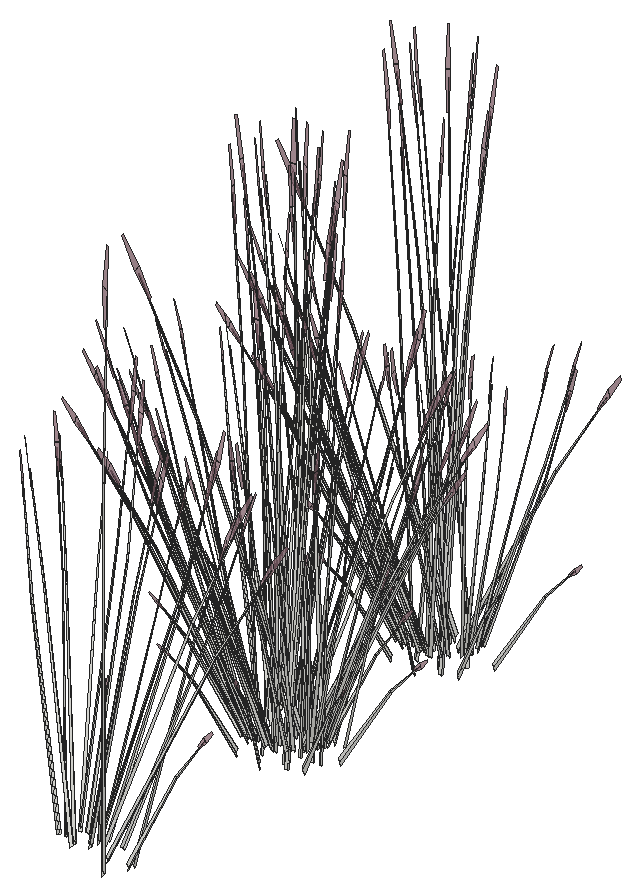
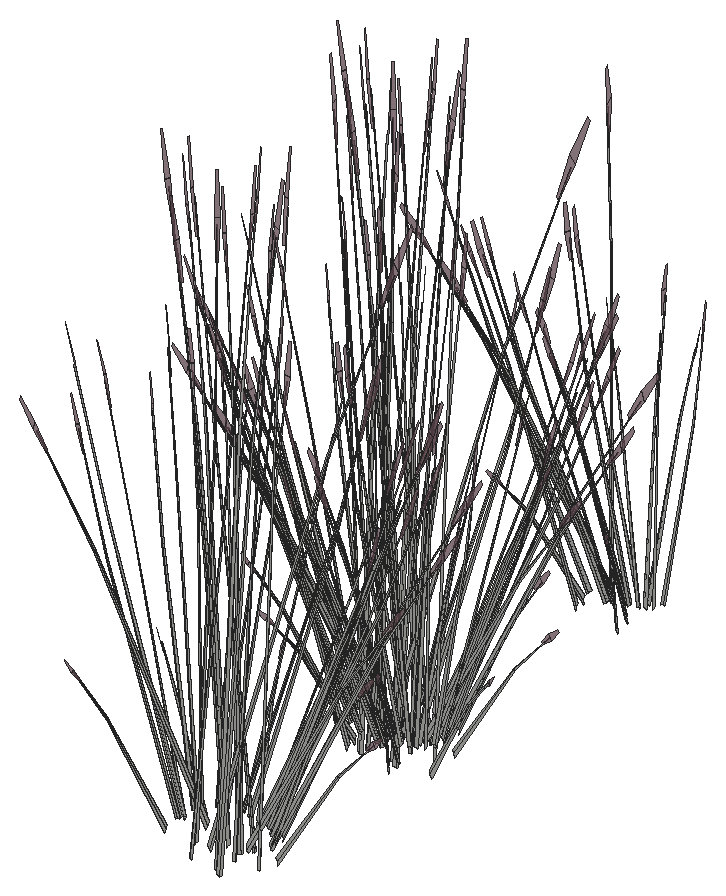
# SketchUp Ruby script. Lengths in inches.
U = 1.inch
M = Sketchup.active_model
def pt(a) = Geom::Point3d.new(a.map { |v| v * U })
def face(e, loops, mat)
  f = e.add_face(loops[0].map { |a| pt(a) })
  loops[1..].each { |l| e.add_face(l.map { |a| pt(a) }).erase! }
  f.material = f.back_material = mat if mat
  f
end
# faces: each face lists its corners as indices into pts; further lists are holes
def faces(e, pts, list, mat = nil) = list.each { |f| face(e, (f[0].is_a?(Array) ? f : [f]).map { |l| l.map { |i| pts[i] } }, mat) }
# xy, xz, yz: faces in a plane at the given z, y or x. An outline is a flat list of corners, or four numbers for a rectangle; further outlines are holes
def ring(l) = l.size == 4 ? [[l[0], l[1]], [l[2], l[1]], [l[2], l[3]], [l[0], l[3]]] : l.each_slice(2).to_a
def flat(e, list, mat, &to3) = list.each { |f| face(e, (f[0].is_a?(Array) ? f : [f]).map { |l| ring(l).map { |u, v| to3.(u, v) } }, mat) }
def xy(e, z, list, mat = nil) = flat(e, list, mat) { |x, y| [x, y, z] }
def xz(e, y, list, mat = nil) = flat(e, list, mat) { |x, z| [x, y, z] }
def yz(e, x, list, mat = nil) = flat(e, list, mat) { |y, z| [x, y, z] }
def lines(e, pts, list) = list.each { |a, b| e.add_line(pt(pts[a]), pt(pts[b])) }
# prism: a flat outline (further loops are holes) pulled along v
def prism(e, loops, v, mat = nil)
  f = face(e, loops, mat); d = Geom::Vector3d.new(v.map { |x| x * U })
  f.pushpull(f.normal.samedirection?(d) ? d.length : -d.length)
end
def box(e, o, s, mat = nil) = prism(e, [[o, [o[0] + s[0], o[1], o[2]], [o[0] + s[0], o[1] + s[1], o[2]], [o[0], o[1] + s[1], o[2]]]], [0, 0, s[2]], mat)
def at(x, y, z, deg = 0) = Geom::Transformation.translation(pt([x, y, z])) * Geom::Transformation.rotation(ORIGIN, Z_AXIS, deg.degrees)
def axes(o, x, y, z) = Geom::Transformation.new([*x, 0, *y, 0, *z, 0, *pt(o).to_a, 1])
def part(name) = M.definitions.add(name)
# library, detail: a bought-in or finely detailed component or shape, given as its bounding box
def library(name, o, s) = part(name).tap { |d| box(d.entities, o, s) }
def detail(e, o, s) = box(e.add_group.entities, o, s)
def put(e, d, t, mat = nil) = e.add_instance(d, t).tap { |i| i.material = mat if mat }
def group(e, t, mat = nil) = e.add_group.tap { |g| g.transformation = t; g.material = mat if mat }.entities
root = M.entities
M.materials.add("LightPink_Translucent").color = [144, 107, 117]
M.materials["LightPink_Translucent"].alpha = 0.75
c1 = part("blade")
p = [[2.15,0.21,22],[0,0.17,0],[0.09,0.45,0],[2.18,0.31,22],[2.29,0.31,22],[0.38,0.45,0],
  [2.48,0.24,33],[2.49,0.24,33],[2.48,0.22,33]]
faces(c1.entities,p,[[0,1,2,3],[4,5,2,3],[6,3,4,7],[8,0,3,6]])
c2 = part("seeds")
p = [[0.3,-0.1,1.38],[-0.01,-0.03,1.59],[-0.01,-0.03,0.03],[0.14,-0.07,-0.07],[0.29,-0.03,3],[0.15,0.01,3.11]]
faces(c2.entities,p,[[0,1,2,3],[1,0,4,5]],"LightPink_Translucent")
c3 = part("blade with seeds")
put(c3.entities,c1,at(0,0,0))
put(c3.entities,c2,axes([2.4,0.25,30.99],[1.5799,-0.05474,1.17369],[-0.12525,1.92788,0.29478],[-0.07173,-0.02425,1.56792]))
put(root,c3,axes([668.72,239.06,513.76],[-0.56631,0.0816,-0.29394],[-0.14954,-0.46647,0.37948],[-0.16229,0.12529,0.72609]))
put(root,c3,axes([672.9,238.78,513.22],[-0.24166,-0.09837,1.42242],[0.50011,-0.41269,0.11501],[0.3117,0.18617,0.60807]))
put(root,c3,axes([673.79,239.9,512.3],[-0.36631,-0.16417,0.95334],[0.47299,-0.16681,0.70045],[0.12758,0.1413,0.20998]))
put(root,c3,axes([669.7,238.6,513.22],[0.1625,-0.17544,1.42242],[0.41029,0.47354,0.11501],[-0.28141,0.21565,0.60807]))
put(root,c3,axes([669.1875,239.11,513.89],[0.16713,0.52135,-0.42412],[-0.63294,0.0912,-0.32852],[-0.18138,0.14003,0.81151]))
put(root,c3,axes([672.9,238.06,512.36],[-0.01777,-0.53759,1.17256],[0.80434,0.13935,0.49647],[-0.19024,0.29416,1.1068]))
put(root,c3,axes([672.96,240.13,513.89],[0.64198,-0.13573,-0.42412],[0.1123,0.514,-0.32852],[0.17243,0.1473,0.81151]))
put(root,c3,axes([673.85,240.65,512.21],[-0.4172,-0.01791,0.872],[0.27552,-0.38032,0.48145],[0.16481,0.13512,0.68401]))
put(root,c3,axes([669.58,239.03,513.22],[0.12114,-0.19625,1.42242],[0.50818,0.40613,0.11501],[-0.22925,0.25313,0.60807]))
put(root,c3,axes([669.72,240.14,513.76],[-0.4402,0.30062,-0.29394],[-0.41671,-0.34326,0.37948],[-0.0634,0.1744,0.72609]))
put(root,c3,axes([670,241.31,512.3],[-0.01684,-0.3395,0.95334],[0.42072,0.24214,0.70045],[-0.08274,0.16182,0.20998]))
put(root,c3,axes([670.16,240,514.15],[0.46573,0.38364,-0.47077],[-0.49199,0.33598,-0.36465],[-0.07086,0.19492,0.90078]))
put(root,c3,axes([671.54,240.37,513.89],[0.63954,0.14313,-0.42412],[-0.21921,0.49074,-0.32852],[0.05864,0.19758,0.81151]))
put(root,c3,axes([671.9,239.35,513.22],[-0.14872,-0.18332,1.42242],[0.6872,-0.15433,0.11501],[0.15531,0.28779,0.60807]))
put(root,c3,axes([671.25,240.67,513.76],[-0.19614,0.43908,-0.29394],[-0.57222,-0.12807,0.37948],[0.05247,0.17678,0.72609]))
put(root,c3,axes([670.01,239.82,514.43],[-0.01693,0.52814,-0.65454],[-0.71285,-0.03547,0.07899],[-0.07523,0.22375,0.92591]))
put(root,c3,axes([670.6875,239.45,513.22],[-0.01592,-0.21915,1.42242],[0.69015,0.14538,0.11501],[-0.04269,0.3123,0.60807]))
put(root,c3,axes([671.3,240.27,514.13],[0.31051,0.46426,-0.58968],[-0.63919,0.25873,0.07116],[0.07261,0.22432,0.83415]))
put(root,c3,axes([669.77,240.5625,512.79],[0.01429,-0.29475,1.28107],[0.64291,0.15569,0.17703],[-0.0557,0.31414,0.60492]))
put(root,c3,axes([670.27,257.61,513.22],[0.14872,0.18332,1.42242],[-0.6872,0.15433,0.11501],[-0.15531,-0.28779,0.60807]))
put(root,c3,axes([672.1,257.75,514.13],[-0.31051,-0.46426,-0.58968],[0.63919,-0.25873,0.07116],[-0.07261,-0.22432,0.83415]))
put(root,c3,axes([673.39,258.2,514.13],[0.01693,-0.52814,-0.58968],[0.71285,0.03547,0.07116],[0.07523,-0.22375,0.83415]))
put(root,c3,axes([672.16,257.35,513.76],[0.19614,-0.43908,-0.29394],[0.57222,0.12807,0.37948],[-0.05247,-0.17678,0.72609]))
put(root,c3,axes([672.59,257.93,513.22],[-0.12114,0.19625,1.42242],[-0.50818,-0.40613,0.11501],[0.22925,-0.25313,0.60807]))
put(root,c3,axes([671.87,257.65,513.89],[-0.63954,-0.14313,-0.42412],[0.21921,-0.49074,-0.32852],[-0.05864,-0.19758,0.81151]))
put(root,c3,axes([672.26,256.43,512.3],[0.08346,0.33295,0.95334],[-0.46298,-0.1844,0.70045],[0.04982,-0.17048,0.20998]))
put(root,c3,axes([673.25,258.03,513.89],[-0.46573,-0.38364,-0.42412],[0.49199,-0.33598,-0.32852],[0.07086,-0.19492,0.81151]))
put(root,c3,axes([673.69,257.88,513.76],[0.4402,-0.30062,-0.29394],[0.41671,0.34326,0.37948],[0.0634,-0.1744,0.72609]))
put(root,c3,axes([669.88,256.83,512.3],[0.33937,0.19872,0.95334],[-0.49424,0.11946,0.70045],[-0.10575,-0.15273,0.20998]))
put(root,c3,axes([670.7,257.88,514.13],[-0.55475,-0.27598,-0.58968],[0.39425,-0.48361,0.07116],[-0.20099,-0.16478,0.83415]))
put(root,c3,axes([670.51,257.51,513.76],[-0.10048,-0.4599,-0.29394],[0.5744,-0.12144,0.37948],[-0.15428,-0.13179,0.72609]))
put(root,c3,axes([669.27,258.18,513.22],[0.24166,0.09837,1.42242],[-0.50011,0.41269,0.11501],[-0.3117,-0.18617,0.60807]))
put(root,c3,axes([670.44,257.89,513.89],[-0.64198,0.13573,-0.42412],[-0.1123,-0.514,-0.32852],[-0.17243,-0.1473,0.81151]))
put(root,c3,axes([674.23,259.12,514.13],[0.33983,-0.45051,-0.58968],[0.59551,0.32017,0.07116],[0.20291,-0.16322,0.83415]))
put(root,c3,axes([674.21,258.91,513.89],[-0.16713,-0.52135,-0.42412],[0.63294,-0.0912,-0.32852],[0.18138,-0.14003,0.81151]))
put(root,c3,axes([672.03,261,512.76],[0.56221,0.23024,1.25546],[-0.55078,0.49601,0.49647],[-0.2467,-0.29398,1.05249]))
put(root,c3,axes([674.99,257.87,512.3],[-0.2167,0.29065,0.95334],[-0.18626,-0.3905,0.70045],[0.17898,-0.09785,0.20998]))
put(root,c3,axes([674.68,258.96,513.76],[0.56631,-0.0816,-0.29394],[0.14954,0.46647,0.37948],[0.16229,-0.12529,0.72609]))
put(root,c3,axes([669.18,258.32,513.76],[-0.37017,-0.35748,-0.29394],[0.42268,-0.3384,0.37948],[-0.21476,-0.05149,0.72609]))
put(root,c3,axes([669.57,258.5625,514.13],[-0.65035,-0.01375,-0.58968],[0.04368,-0.5789,0.07116],[-0.27552,-0.06109,0.83415]))
put(root,c3,axes([669.35,258.68,513.89],[-0.47241,0.37822,-0.42412],[-0.41372,-0.39954,-0.32852],[-0.24002,-0.05755,0.81151]))
put(root,c3,axes([668.29,259.18,512.3],[0.41536,-0.04086,0.95334],[-0.26347,0.35999,0.70045],[-0.20525,-0.054,0.20998]))
put(root,c3,axes([671.22,259.51,512.26],[-0.70648,0.03525,0.37133],[-0.06389,-0.58508,-0.17871],[0.12647,-0.0593,1.19224]))
put(root,c3,axes([669.4,259.9375,512.06],[0,0.57097,0.4121],[-0.72788,0,0],[0,-0.13004,1.30728]))
put(root,c3,axes([674.51,260.07,513.89],[0.17625,-0.51936,-0.42412],[0.60429,0.17802,-0.32852],[0.2433,-0.04762,0.81151]))
put(root,c3,axes([668.76,259.08,513.22],[0.26985,-0.01293,1.42242],[-0.17902,0.56047,0.11501],[-0.38456,-0.03467,0.60807]))
put(root,c3,axes([671.06,260.23,512.26],[-0.31565,0.51449,0.37133],[-0.65588,-0.24761,-0.17871],[0,-0.1186,1.19224]))
put(root,c3,axes([673.2,258.25,512.06],[-0.60889,-0.28548,0.4121],[0.36394,-0.51192,0],[0.13868,0.06502,1.30728]))
put(root,c3,axes([674.39,260.26,514.13],[0.57168,-0.25217,-0.58968],[0.3186,0.51908,0.07116],[0.27622,-0.05897,0.83415]))
put(root,c3,axes([670.89,258.51,512.05],[-0.18794,0.56744,0.14643],[-0.68774,-0.16058,0.29122],[0.1188,-0.00276,1.33138]))
put(root,c3,axes([672.07,259.27,512.26],[-0.39083,-0.47924,0.37133],[0.59199,-0.33747,-0.17871],[0.12647,0.0593,1.19224]))
put(root,c3,axes([670.83,261.43,512.05],[0.6991,-0.15154,0.14643],[0.17263,0.56398,0.29122],[-0.06235,-0.08217,1.33138]))
put(root,c3,axes([674.88,260.3,513.76],[0.54068,0.15928,-0.29394],[-0.1577,0.46469,0.37948],[0.21769,-0.04261,0.72609]))
put(root,c3,axes([668.52,259.5625,513.76],[-0.54068,-0.15928,-0.29394],[0.1577,-0.46469,0.37948],[-0.21769,0.04261,0.72609]))
put(root,c3,axes([672.97,258.54,512.05],[-0.6991,0.15154,0.14643],[-0.17263,-0.56398,0.29122],[0.06235,0.08217,1.33138]))
put(root,c3,axes([673.41,259.73,513.22],[-0.26985,0.01293,1.42242],[0.17902,-0.56047,0.11501],[0.38456,0.03467,0.60807]))
put(root,c3,axes([672.91,261.47,512.05],[0.18794,-0.56744,0.14643],[0.68774,0.16058,0.29122],[-0.1188,0.00276,1.33138]))
put(root,c3,axes([670.17,259.49,512.77],[0.18493,-0.0826,1.46963],[0.06377,0.5767,0.11501],[-0.40056,0.07652,0.52526]))
put(root,c3,axes([673.98,260.02,512.05],[-0.51116,-0.4159,0.14643],[0.51512,-0.4034,0.29122],[-0.05645,0.08494,1.33138]))
put(root,c3,axes([676.03,260.4,512.3],[-0.40197,0.09426,0.95334],[0.18921,-0.38956,0.70045],[0.21325,0.02666,0.20998]))
put(root,c3,axes([670.6,261.72,512.06],[0.60889,0.28548,0.4121],[-0.36394,0.51192,0],[-0.13868,-0.06502,1.30728]))
put(root,c3,axes([672.75,259.75,512.26],[0.31565,-0.51449,0.37133],[0.65588,0.24761,-0.17871],[0,0.1186,1.19224]))
put(root,c3,axes([668.89,259.8,513.89],[-0.17625,0.51936,-0.42412],[-0.60429,-0.17802,-0.32852],[-0.2433,0.04762,0.81151]))
put(root,c3,axes([675.33,261.6,513.26],[-0.12452,-0.47997,-0.02898],[0.58854,-0.11034,-0.1314],[0.1229,0.03043,0.43341]))
put(root,c3,axes([674.4,260.03,512.06],[0,-0.57097,0.4121],[0.72788,0,0],[0,0.13004,1.30728]))
put(root,c3,axes([672.58,260.46,512.26],[0.70648,-0.03525,0.37133],[0.06389,0.58508,-0.17871],[-0.12647,0.0593,1.19224]))
put(root,c3,axes([668.875,260.07,513.22],[0.22574,-0.12077,1.42242],[0.19004,0.55807,0.11501],[-0.35439,0.12613,0.60807]))
put(root,c3,axes([673.83,261.31,514.13],[0.65035,0.01375,-0.58968],[-0.04368,0.5789,0.07116],[0.27552,0.06109,0.83415]))
put(root,c3,axes([673.1,261.77,512.06],[0.60889,-0.28548,0.4121],[0.36394,0.51192,0],[-0.13868,0.06502,1.30728]))
put(root,c3,axes([667.7,262.02,512.3],[0.27113,-0.25877,0.95334],[0.10699,0.40966,0.70045],[-0.19594,0.07335,0.20998]))
put(root,c3,axes([674.23,261.54,513.76],[0.37017,0.35748,-0.29394],[-0.42268,0.3384,0.37948],[0.21476,0.05149,0.72609]))
put(root,c3,axes([668.72,260.9,513.76],[-0.56631,0.0816,-0.29394],[-0.14954,-0.46647,0.37948],[-0.16229,0.12529,0.72609]))
put(root,c3,axes([672.9,260.63,513.22],[-0.24166,-0.09837,1.42242],[0.50011,-0.41269,0.11501],[0.3117,0.18617,0.60807]))
put(root,c3,axes([673.79,261.75,512.3],[-0.36631,-0.16417,0.95334],[0.47299,-0.16681,0.70045],[0.12758,0.1413,0.20998]))
put(root,c3,axes([669.7,260.44,513.22],[0.1625,-0.17544,1.42242],[0.41029,0.47354,0.11501],[-0.28141,0.21565,0.60807]))
put(root,c3,axes([669.1875,260.96,513.89],[0.16713,0.52135,-0.42412],[-0.63294,0.0912,-0.32852],[-0.18138,0.14003,0.81151]))
put(root,c3,axes([672.9,259.9,512.36],[-0.01777,-0.53759,1.17256],[0.80434,0.13935,0.49647],[-0.19024,0.29416,1.1068]))
put(root,c3,axes([672.96,261.97,513.89],[0.64198,-0.13573,-0.42412],[0.1123,0.514,-0.32852],[0.17243,0.1473,0.81151]))
put(root,c3,axes([673.85,262.5,512.21],[-0.4172,-0.01791,0.872],[0.27552,-0.38032,0.48145],[0.16481,0.13512,0.68401]))
put(root,c3,axes([669.58,260.875,513.22],[0.12114,-0.19625,1.42242],[0.50818,0.40613,0.11501],[-0.22925,0.25313,0.60807]))
put(root,c3,axes([669.72,261.98,513.76],[-0.4402,0.30062,-0.29394],[-0.41671,-0.34326,0.37948],[-0.0634,0.1744,0.72609]))
put(root,c3,axes([670,263.15,512.3],[-0.01684,-0.3395,0.95334],[0.42072,0.24214,0.70045],[-0.08274,0.16182,0.20998]))
put(root,c3,axes([670.16,261.84,514.15],[0.46573,0.38364,-0.47077],[-0.49199,0.33598,-0.36465],[-0.07086,0.19492,0.90078]))
put(root,c3,axes([671.54,262.21,513.89],[0.63954,0.14313,-0.42412],[-0.21921,0.49074,-0.32852],[0.05864,0.19758,0.81151]))
put(root,c3,axes([671.9,261.2,513.22],[-0.14872,-0.18332,1.42242],[0.6872,-0.15433,0.11501],[0.15531,0.28779,0.60807]))
put(root,c3,axes([671.25,262.51,513.76],[-0.19614,0.43908,-0.29394],[-0.57222,-0.12807,0.37948],[0.05247,0.17678,0.72609]))
put(root,c3,axes([670.01,261.67,514.43],[-0.01693,0.52814,-0.65454],[-0.71285,-0.03547,0.07899],[-0.07523,0.22375,0.92591]))
put(root,c3,axes([670.6875,261.29,513.22],[-0.01592,-0.21915,1.42242],[0.69015,0.14538,0.11501],[-0.04269,0.3123,0.60807]))
put(root,c3,axes([671.3,262.12,514.13],[0.31051,0.46426,-0.58968],[-0.63919,0.25873,0.07116],[0.07261,0.22432,0.83415]))
put(root,c3,axes([669.77,262.41,512.79],[0.01429,-0.29475,1.28107],[0.64291,0.15569,0.17703],[-0.0557,0.31414,0.60492]))
put(root,c3,axes([670.27,274.47,513.22],[0.14872,0.18332,1.42242],[-0.6872,0.15433,0.11501],[-0.15531,-0.28779,0.60807]))
put(root,c3,axes([672.1,274.61,514.13],[-0.31051,-0.46426,-0.58968],[0.63919,-0.25873,0.07116],[-0.07261,-0.22432,0.83415]))
put(root,c3,axes([673.39,275.06,514.13],[0.01693,-0.52814,-0.58968],[0.71285,0.03547,0.07116],[0.07523,-0.22375,0.83415]))
put(root,c3,axes([672.16,274.21,513.76],[0.19614,-0.43908,-0.29394],[0.57222,0.12807,0.37948],[-0.05247,-0.17678,0.72609]))
put(root,c3,axes([672.59,274.79,513.22],[-0.12114,0.19625,1.42242],[-0.50818,-0.40613,0.11501],[0.22925,-0.25313,0.60807]))
put(root,c3,axes([671.87,274.51,513.89],[-0.63954,-0.14313,-0.42412],[0.21921,-0.49074,-0.32852],[-0.05864,-0.19758,0.81151]))
put(root,c3,axes([672.26,273.28,512.3],[0.08346,0.33295,0.95334],[-0.46298,-0.1844,0.70045],[0.04982,-0.17048,0.20998]))
put(root,c3,axes([673.25,274.89,513.89],[-0.46573,-0.38364,-0.42412],[0.49199,-0.33598,-0.32852],[0.07086,-0.19492,0.81151]))
put(root,c3,axes([673.69,274.74,513.76],[0.4402,-0.30062,-0.29394],[0.41671,0.34326,0.37948],[0.0634,-0.1744,0.72609]))
put(root,c3,axes([669.88,273.68,512.3],[0.33937,0.19872,0.95334],[-0.49424,0.11946,0.70045],[-0.10575,-0.15273,0.20998]))
put(root,c3,axes([670.7,274.74,514.13],[-0.55475,-0.27598,-0.58968],[0.39425,-0.48361,0.07116],[-0.20099,-0.16478,0.83415]))
put(root,c3,axes([670.51,274.37,513.76],[-0.10048,-0.4599,-0.29394],[0.5744,-0.12144,0.37948],[-0.15428,-0.13179,0.72609]))
put(root,c3,axes([669.27,275.04,513.22],[0.24166,0.09837,1.42242],[-0.50011,0.41269,0.11501],[-0.3117,-0.18617,0.60807]))
put(root,c3,axes([670.44,274.75,513.89],[-0.64198,0.13573,-0.42412],[-0.1123,-0.514,-0.32852],[-0.17243,-0.1473,0.81151]))
put(root,c3,axes([674.23,275.98,514.13],[0.33983,-0.45051,-0.58968],[0.59551,0.32017,0.07116],[0.20291,-0.16322,0.83415]))
put(root,c3,axes([674.21,275.77,513.89],[-0.16713,-0.52135,-0.42412],[0.63294,-0.0912,-0.32852],[0.18138,-0.14003,0.81151]))
put(root,c3,axes([672.03,277.86,512.76],[0.56221,0.23024,1.25546],[-0.55078,0.49601,0.49647],[-0.2467,-0.29398,1.05249]))
put(root,c3,axes([674.99,274.73,512.3],[-0.2167,0.29065,0.95334],[-0.18626,-0.3905,0.70045],[0.17898,-0.09785,0.20998]))
put(root,c3,axes([674.68,275.82,513.76],[0.56631,-0.0816,-0.29394],[0.14954,0.46647,0.37948],[0.16229,-0.12529,0.72609]))
put(root,c3,axes([669.18,275.18,513.76],[-0.37017,-0.35748,-0.29394],[0.42268,-0.3384,0.37948],[-0.21476,-0.05149,0.72609]))
put(root,c3,axes([669.57,275.42,514.13],[-0.65035,-0.01375,-0.58968],[0.04368,-0.5789,0.07116],[-0.27552,-0.06109,0.83415]))
put(root,c3,axes([669.35,275.54,513.89],[-0.47241,0.37822,-0.42412],[-0.41372,-0.39954,-0.32852],[-0.24002,-0.05755,0.81151]))
put(root,c3,axes([668.29,276.04,512.3],[0.41536,-0.04086,0.95334],[-0.26347,0.35999,0.70045],[-0.20525,-0.054,0.20998]))
put(root,c3,axes([671.22,276.37,512.26],[-0.70648,0.03525,0.37133],[-0.06389,-0.58508,-0.17871],[0.12647,-0.0593,1.19224]))
put(root,c3,axes([669.4,276.8,512.06],[0,0.57097,0.4121],[-0.72788,0,0],[0,-0.13004,1.30728]))
put(root,c3,axes([674.51,276.93,513.89],[0.17625,-0.51936,-0.42412],[0.60429,0.17802,-0.32852],[0.2433,-0.04762,0.81151]))
put(root,c3,axes([668.76,275.94,513.22],[0.26985,-0.01293,1.42242],[-0.17902,0.56047,0.11501],[-0.38456,-0.03467,0.60807]))
put(root,c3,axes([671.06,277.09,512.26],[-0.31565,0.51449,0.37133],[-0.65588,-0.24761,-0.17871],[0,-0.1186,1.19224]))
put(root,c3,axes([673.2,275.11,512.06],[-0.60889,-0.28548,0.4121],[0.36394,-0.51192,0],[0.13868,0.06502,1.30728]))
put(root,c3,axes([674.39,277.11,514.13],[0.57168,-0.25217,-0.58968],[0.3186,0.51908,0.07116],[0.27622,-0.05897,0.83415]))
put(root,c3,axes([670.89,275.37,512.05],[-0.18794,0.56744,0.14643],[-0.68774,-0.16058,0.29122],[0.1188,-0.00276,1.33138]))
put(root,c3,axes([672.07,276.13,512.26],[-0.39083,-0.47924,0.37133],[0.59199,-0.33747,-0.17871],[0.12647,0.0593,1.19224]))
put(root,c3,axes([670.83,278.29,512.05],[0.6991,-0.15154,0.14643],[0.17263,0.56398,0.29122],[-0.06235,-0.08217,1.33138]))
put(root,c3,axes([674.88,277.16,513.76],[0.54068,0.15928,-0.29394],[-0.1577,0.46469,0.37948],[0.21769,-0.04261,0.72609]))
put(root,c3,axes([668.52,276.42,513.76],[-0.54068,-0.15928,-0.29394],[0.1577,-0.46469,0.37948],[-0.21769,0.04261,0.72609]))
put(root,c3,axes([672.97,275.4,512.05],[-0.6991,0.15154,0.14643],[-0.17263,-0.56398,0.29122],[0.06235,0.08217,1.33138]))
put(root,c3,axes([673.41,276.59,513.22],[-0.26985,0.01293,1.42242],[0.17902,-0.56047,0.11501],[0.38456,0.03467,0.60807]))
put(root,c3,axes([672.91,278.32,512.05],[0.18794,-0.56744,0.14643],[0.68774,0.16058,0.29122],[-0.1188,0.00276,1.33138]))
put(root,c3,axes([670.17,276.35,512.77],[0.18493,-0.0826,1.46963],[0.06377,0.5767,0.11501],[-0.40056,0.07652,0.52526]))
put(root,c3,axes([673.98,276.875,512.05],[-0.51116,-0.4159,0.14643],[0.51512,-0.4034,0.29122],[-0.05645,0.08494,1.33138]))
put(root,c3,axes([676.03,277.26,512.3],[-0.40197,0.09426,0.95334],[0.18921,-0.38956,0.70045],[0.21325,0.02666,0.20998]))
put(root,c3,axes([670.6,278.58,512.06],[0.60889,0.28548,0.4121],[-0.36394,0.51192,0],[-0.13868,-0.06502,1.30728]))
